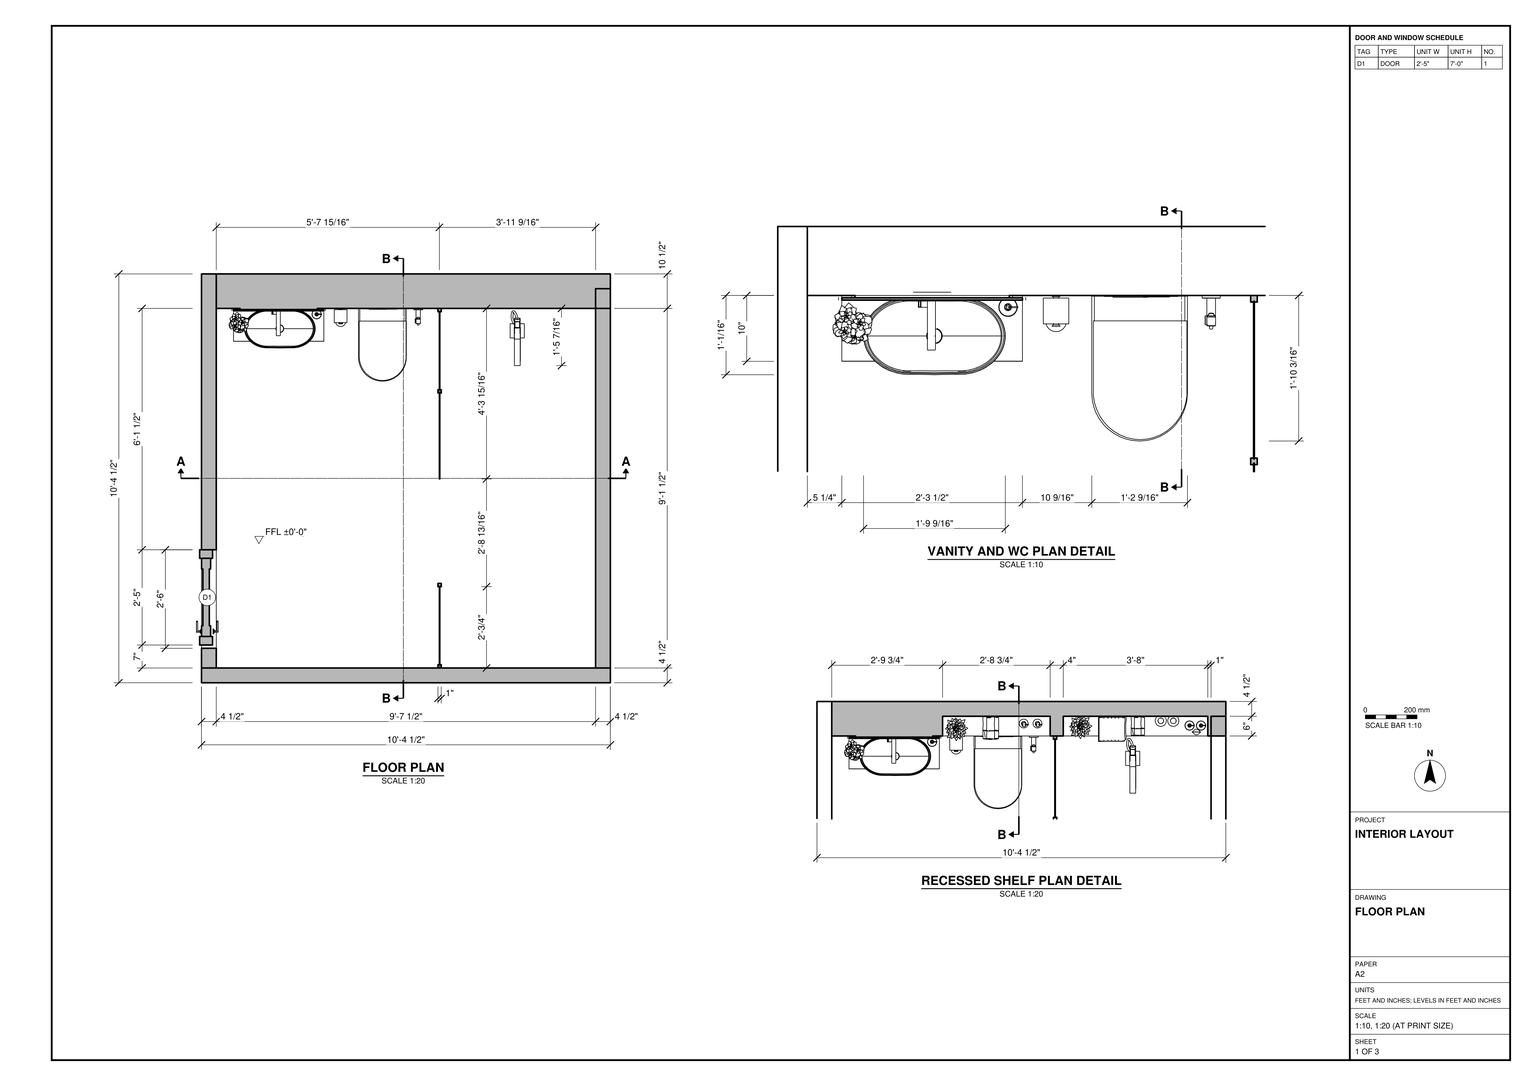
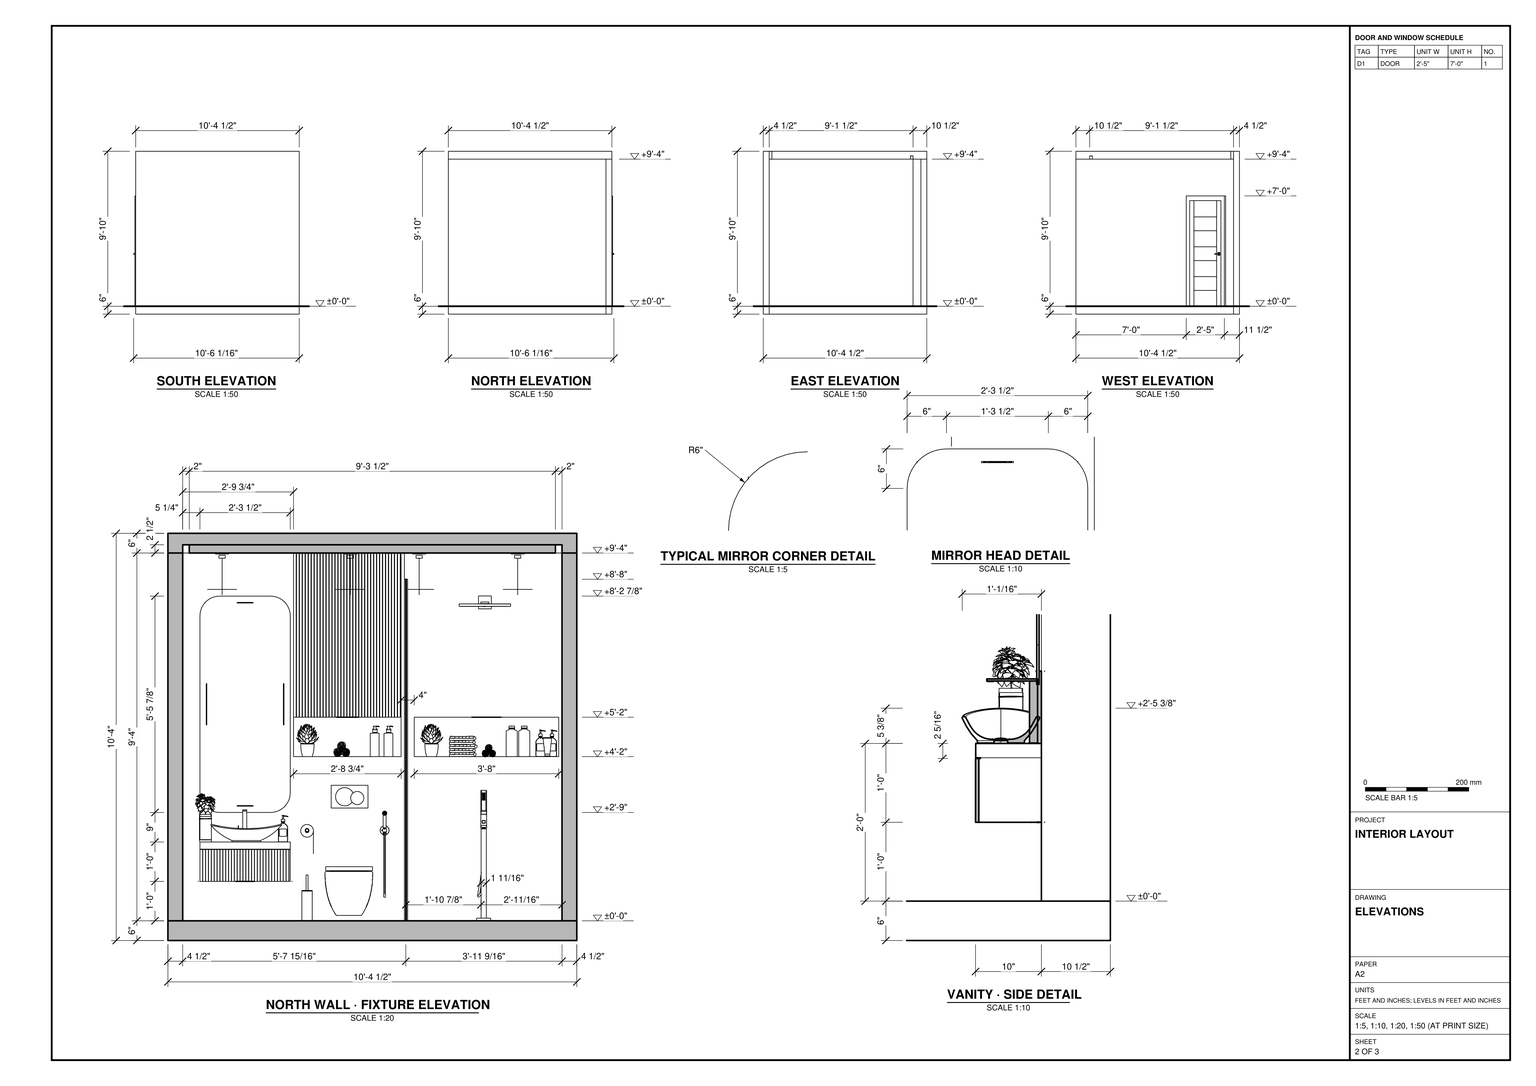
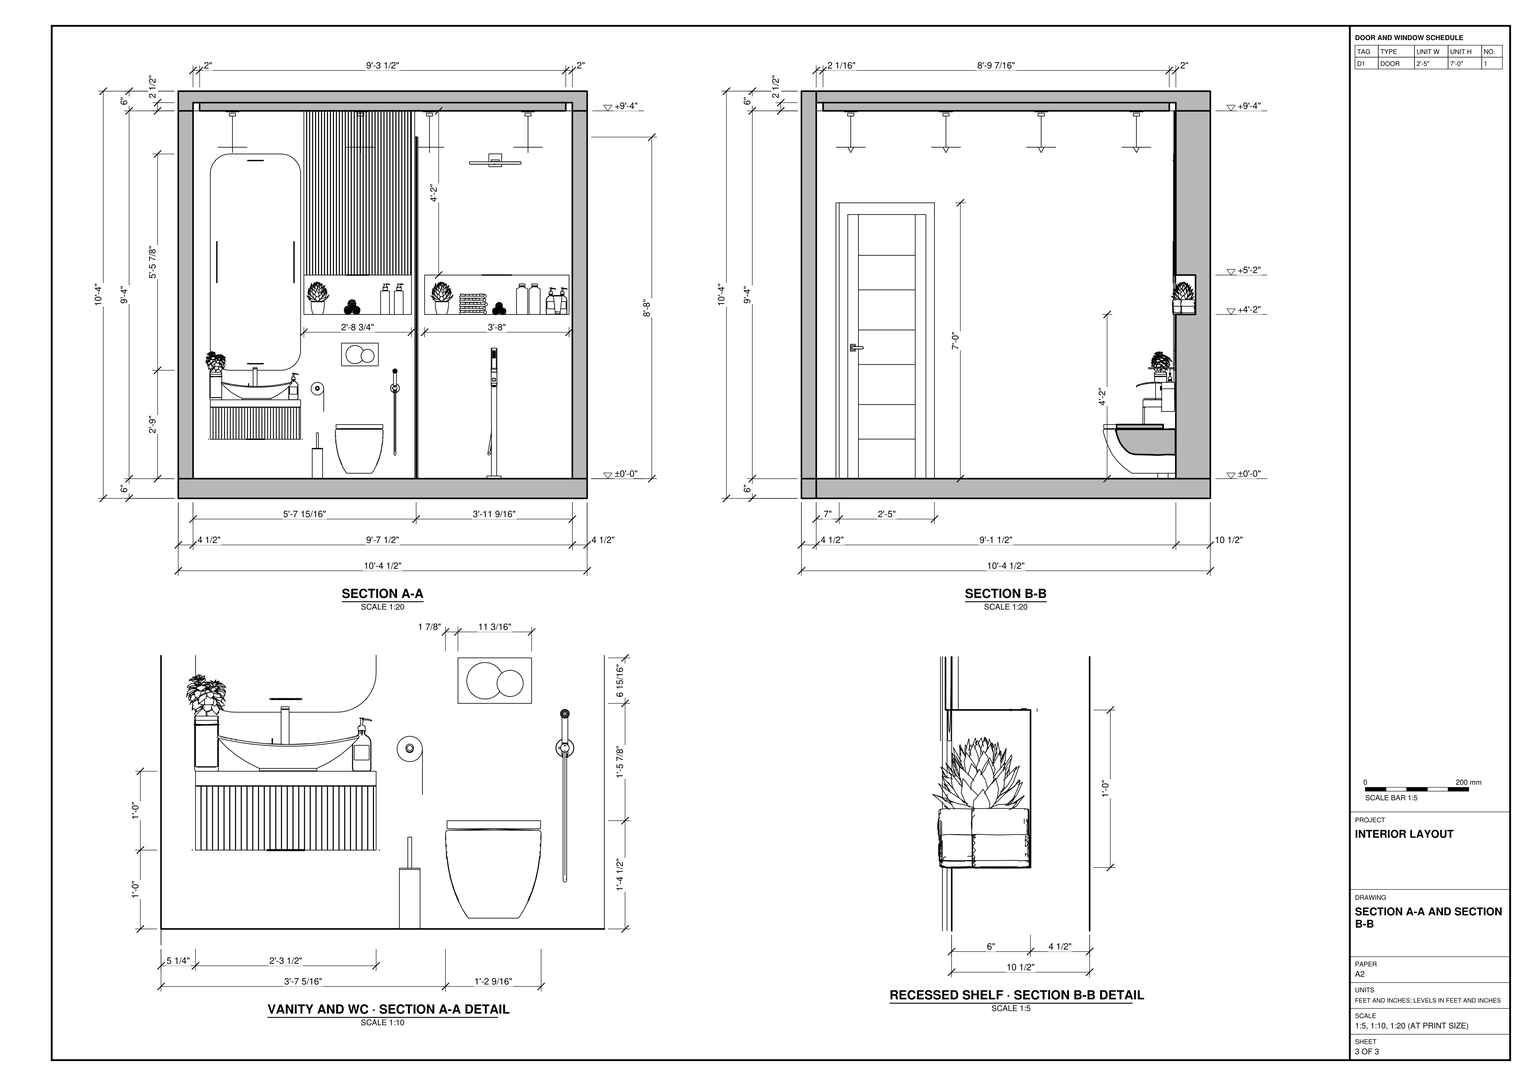
Use the plan, elevations, sections and details in task_files/diagram_01.pdf to build the bathroom in SketchUp. Work in feet and inches. Make the overall model 10'-6 1/16" along X, 10'-4 1/2" along Y and 10'-4" high, with the finished floor at ±0'-0".

Model the floor slab, perimeter walls and ceiling assembly in section. Use the wall thicknesses shown in plan: the north fixture wall is thicker than the other walls to accommodate the recessed shelves. Include the door near the south end of the west wall and a window unit.

Use the north wall elevation to arrange the fixtures. Place the floating vanity with its ribbed front, basin and tap beneath the tall, rounded-corner mirror. Set the wall-hung toilet beside the vanity, with its flush plate above. Model the shelf recesses over the toilet and in the shower area, including the vertically ribbed panel above the toilet recess. On the east side, place the shower fittings behind the glass screens and leave the passage between the screens open as shown in plan. Plants, toiletries, lights and other loose or decorative items may be any suitable library components placed as shown.

Keep the walls, slabs, ceiling assembly and individual fixtures and joinery pieces in separate groups or components. Use components for repeated parts. Save one SketchUp model as output_files/bathroom_with_a_floating_vanity_and_screened_shower.skp.

# SketchUp Ruby script. Lengths in inches.
U = 1.inch
M = Sketchup.active_model
def pt(a) = Geom::Point3d.new(a.map { |v| v * U })
def face(e, loops, mat)
  f = e.add_face(loops[0].map { |a| pt(a) })
  loops[1..].each { |l| e.add_face(l.map { |a| pt(a) }).erase! }
  f.material = f.back_material = mat if mat
  f
end
# faces: each face lists its corners as indices into pts; further lists are holes
def faces(e, pts, list, mat = nil) = list.each { |f| face(e, (f[0].is_a?(Array) ? f : [f]).map { |l| l.map { |i| pts[i] } }, mat) }
# xy, xz, yz: faces in a plane at the given z, y or x. An outline is a flat list of corners, or four numbers for a rectangle; further outlines are holes
def ring(l) = l.size == 4 ? [[l[0], l[1]], [l[2], l[1]], [l[2], l[3]], [l[0], l[3]]] : l.each_slice(2).to_a
def flat(e, list, mat, &to3) = list.each { |f| face(e, (f[0].is_a?(Array) ? f : [f]).map { |l| ring(l).map { |u, v| to3.(u, v) } }, mat) }
def xy(e, z, list, mat = nil) = flat(e, list, mat) { |x, y| [x, y, z] }
def xz(e, y, list, mat = nil) = flat(e, list, mat) { |x, z| [x, y, z] }
def yz(e, x, list, mat = nil) = flat(e, list, mat) { |y, z| [x, y, z] }
def lines(e, pts, list) = list.each { |a, b| e.add_line(pt(pts[a]), pt(pts[b])) }
# prism: a flat outline (further loops are holes) pulled along v
def prism(e, loops, v, mat = nil)
  f = face(e, loops, mat); d = Geom::Vector3d.new(v.map { |x| x * U })
  f.pushpull(f.normal.samedirection?(d) ? d.length : -d.length)
end
def box(e, o, s, mat = nil) = prism(e, [[o, [o[0] + s[0], o[1], o[2]], [o[0] + s[0], o[1] + s[1], o[2]], [o[0], o[1] + s[1], o[2]]]], [0, 0, s[2]], mat)
def at(x, y, z, deg = 0) = Geom::Transformation.translation(pt([x, y, z])) * Geom::Transformation.rotation(ORIGIN, Z_AXIS, deg.degrees)
def axes(o, x, y, z) = Geom::Transformation.new([*x, 0, *y, 0, *z, 0, *pt(o).to_a, 1])
def part(name) = M.definitions.add(name)
# library, detail: a bought-in or finely detailed component or shape, given as its bounding box
def library(name, o, s) = part(name).tap { |d| box(d.entities, o, s) }
def detail(e, o, s) = box(e.add_group.entities, o, s)
def put(e, d, t, mat = nil) = e.add_instance(d, t).tap { |i| i.material = mat if mat }
def group(e, t, mat = nil) = e.add_group.tap { |g| g.transformation = t; g.material = mat if mat }.entities
root = M.entities
M.materials.add("Generic").color = [129, 129, 129]
M.materials["Generic"].alpha = 0.1
M.materials.add("[Color M00]").color = [255, 255, 255]
M.materials.add("[Metal_Corrogated_Shiny]5").color = [193, 193, 193]
M.materials.add("clear glass1").color = [0, 0, 0]
M.materials["clear glass1"].alpha = 0.1
M.materials.add("lz-doorbrown").color = [51, 28, 20]
M.materials.add("lz-doorhandle").color = [114, 114, 114]
c1 = library("lavabo vasque Villeroy",[-11.67,-6.38,0],[23.35,12.76,5.76])
c2 = library("Toilet accessory set",[0,0,0],[28.35,5.51,33.44])
c3 = library("Wall-hung toilet",[0,-0.05,1.64],[14.57,22.16,39.63])
c4 = library("Shower Bath",[-222.28,-28.8,6],[84.83,24.29,98.92])
c5 = library("Potted Basil 50-07",[-3.85,-3.53,0.03],[7.56,8,18.65])
c6 = library("Potted Plant 50-23",[-3.4,-3.5,0],[6.8,7,9.93])
c7 = library("Folded towel stack",[36.8,35.16,1.14],[12.05,13.22,9.67])
c8 = library("Rolled towel stack",[-0.87,0,-0.63],[7.91,9.92,7.86])
c9 = part("Door lever handle")
xy(c9.entities,0,[[0,0,1.888,1.971]])
xy(c9.entities,0.197,[[[0,0,1.888,1.971],[0.307,0.321,1.58,1.65]]])
xy(c9.entities,0.394,[[[0.307,0.321,1.58,1.65],[0.954,0.632,0.96,0.632,0.96,1.339,0.954,1.339,0.868,1.328,0.782,1.292,0.709,1.236,0.653,1.162,0.617,1.077,0.605,0.985,0.617,0.894,0.653,0.808,0.709,0.735,0.782,0.678,0.868,0.643]],[0.954,0.632,0.868,0.643,0.782,0.678,0.709,0.735,0.653,0.808,0.617,0.894,0.605,0.985,0.617,1.077,0.653,1.162,0.709,1.236,0.782,1.292,0.868,1.328,0.954,1.339,0.96,1.339,0.96,0.632],[0.96,0.632,1.265,1.339]])
xy(c9.entities,1.181,[[1.265,0.632,1.265,1.339,4.506,1.339,4.592,1.328,4.677,1.292,4.751,1.236,4.807,1.162,4.842,1.077,4.854,0.985,4.842,0.894,4.807,0.808,4.751,0.735,4.677,0.678,4.592,0.643,4.506,0.632]])
xy(c9.entities,1.535,[[0.954,0.632,0.868,0.643,0.782,0.678,0.709,0.735,0.653,0.808,0.617,0.894,0.605,0.985,0.617,1.077,0.653,1.162,0.709,1.236,0.782,1.292,0.868,1.328,0.954,1.339,4.506,1.339,4.592,1.328,4.677,1.292,4.751,1.236,4.807,1.162,4.842,1.077,4.854,0.985,4.842,0.894,4.807,0.808,4.751,0.735,4.677,0.678,4.592,0.643,4.506,0.632]])
xy(c9.entities,1.575,[[0.956,0.671,0.878,0.681,0.802,0.713,0.737,0.763,0.687,0.828,0.656,0.904,0.645,0.985,0.656,1.067,0.687,1.143,0.737,1.208,0.802,1.258,0.878,1.289,0.956,1.3,4.503,1.3,4.581,1.289,4.657,1.258,4.722,1.208,4.772,1.143,4.804,1.067,4.815,0.985,4.804,0.904,4.772,0.828,4.722,0.763,4.657,0.713,4.581,0.681,4.503,0.671]])
xz(c9.entities,0,[[0,0,1.888,0.197]])
xz(c9.entities,0.321,[[0.307,0.197,1.58,0.394]])
xz(c9.entities,0.632,[[0.954,0.394,0.96,1.535],[0.96,0.394,0.96,1.535,4.506,1.535,4.506,1.181,1.265,1.181,1.265,0.394]])
xz(c9.entities,1.339,[[0.954,0.394,0.96,1.535],[0.96,0.394,1.265,0.394,1.265,1.181,4.506,1.181,4.506,1.535,0.96,1.535]])
xz(c9.entities,1.65,[[0.307,0.197,1.58,0.394]])
xz(c9.entities,1.971,[[0,0,1.888,0.197]])
yz(c9.entities,0,[[0,0,1.971,0.197]])
yz(c9.entities,0.307,[[0.321,0.197,1.65,0.394]])
yz(c9.entities,1.265,[[0.632,0.394,1.339,1.181]])
yz(c9.entities,1.58,[[0.321,0.197,1.65,0.394]])
yz(c9.entities,1.888,[[0,0,1.971,0.197]])
p = [[0.782,0.678,1.535],[0.868,0.643,1.535],[0.868,0.643,0.394],[0.782,0.678,0.394],[0.954,0.632,1.535],[0.954,0.632,0.394],
  [0.653,0.808,1.535],[0.709,0.735,1.535],[0.709,0.735,0.394],[0.653,0.808,0.394],[0.617,0.894,1.535],[0.617,0.894,0.394],
  [0.605,0.985,1.535],[0.605,0.985,0.394],[0.617,1.077,1.535],[0.617,1.077,0.394],[0.653,1.162,1.535],[0.653,1.162,0.394],
  [0.782,1.292,1.535],[0.709,1.236,1.535],[0.709,1.236,0.394],[0.782,1.292,0.394],[0.868,1.328,1.535],[0.868,1.328,0.394],
  [0.954,1.339,1.535],[0.954,1.339,0.394],[4.592,0.643,1.535],[4.506,0.632,1.535],[4.506,0.632,1.181],[4.592,0.643,1.181],
  [4.677,0.678,1.535],[4.677,0.678,1.181],[4.751,0.735,1.535],[4.751,0.735,1.181],[4.807,0.808,1.535],[4.807,0.808,1.181],
  [4.842,0.894,1.535],[4.842,0.894,1.181],[4.854,0.985,1.535],[4.854,0.985,1.181],[4.842,1.077,1.535],[4.842,1.077,1.181],
  [4.807,1.162,1.535],[4.807,1.162,1.181],[4.677,1.292,1.535],[4.751,1.236,1.535],[4.751,1.236,1.181],[4.677,1.292,1.181],
  [4.506,1.339,1.535],[4.592,1.328,1.535],[4.592,1.328,1.181],[4.506,1.339,1.181],[0.802,0.713,1.575],[0.878,0.681,1.575],
  [0.956,0.671,1.575],[0.96,0.632,1.535],[0.96,0.671,1.575],[4.503,0.671,1.575],[4.581,0.681,1.575],[4.657,0.713,1.575],
  [0.687,0.828,1.575],[0.737,0.763,1.575],[4.722,0.763,1.575],[4.772,0.828,1.575],[0.656,0.904,1.575],[4.804,0.904,1.575],
  [0.645,0.985,1.575],[4.815,0.985,1.575],[0.656,1.067,1.575],[4.804,1.067,1.575],[0.687,1.143,1.575],[0.737,1.208,1.575],
  [4.772,1.143,1.575],[4.722,1.208,1.575],[0.802,1.258,1.575],[4.657,1.258,1.575],[0.878,1.289,1.575],[0.956,1.3,1.575],
  [0.96,1.3,1.575],[0.96,1.339,1.535],[4.503,1.3,1.575],[4.581,1.289,1.575]]
faces(c9.entities,p,[[0,1,2,3],[1,4,5,2],[6,7,8,9],[7,0,3,8],[10,6,9,11],[12,10,11,13],[14,12,13,15],[16,14,15,17],
  [18,19,20,21],[19,16,17,20],[22,18,21,23],[24,22,23,25],[26,27,28,29],[30,26,29,31],[32,30,31,33],[34,32,33,35],
  [36,34,35,37],[38,36,37,39],[40,38,39,41],[42,40,41,43],[44,45,46,47],[45,42,43,46],[48,49,50,51],[49,44,47,50],
  [0,52,53,1],[1,53,54,4],[55,56,57,27],[54,56,55,4],[27,57,58,26],[26,58,59,30],[6,60,61,7],[7,61,52,0],
  [30,59,62,32],[32,62,63,34],[10,64,60,6],[34,63,65,36],[12,66,64,10],[36,65,67,38],[14,68,66,12],[38,67,69,40],
  [16,70,68,14],[19,71,70,16],[42,72,73,45],[40,69,72,42],[18,74,71,19],[45,73,75,44],[22,76,74,18],[24,77,76,22],
  [78,77,24,79],[79,48,80,78],[49,81,80,48],[44,75,81,49]])
c10 = part("door by lz")
put(c10.entities,c9,axes([9.99,-3.35,36.38],[1,0,0],[0,0,1],[0,-1,0]),"lz-doorhandle")
put(c10.entities,c9,axes([10.03,0.12,36.38],[1,0,0],[0,0,1],[0,1,0]),"lz-doorhandle")
g1 = group(c10.entities,at(5.91,0,0),"lz-doorbrown")
prism(g1,[[[35.43,0,0],[32.26,0,0],[32.26,0,75.4],[3.18,0,75.4],[3.18,0,0],[0,0,0],[0,0,78.74],[35.43,0,78.74]]],[0,-3.9375,0])
g2 = group(c10.entities,at(9.09,-0.59,0),"lz-doorbrown")
xy(g2,0,[[0,-2.76,3.97,-2.76,3.97,-2.36,25.11,-2.36,25.11,-2.76,29.08,-2.76,29.08,0,25.11,0,25.11,-0.39,3.97,-0.39,3.97,0,0,0]])
xy(g2,11.29,[[3.97,-2.36,25.11,-1.97],[3.97,-0.79,25.11,-0.39]])
xy(g2,21.14,[[3.97,-2.36,25.11,-1.97],[3.97,-0.79,25.11,-0.39]])
xy(g2,32.6,[[3.97,-2.36,25.11,-1.97],[3.97,-0.79,25.11,-0.39]])
xy(g2,42.45,[[3.97,-2.36,25.11,-1.97],[3.97,-0.79,25.11,-0.39]])
xy(g2,53.9,[[3.97,-2.36,25.11,-1.97],[3.97,-0.79,25.11,-0.39]])
xy(g2,63.75,[[3.97,-2.36,25.11,-1.97],[3.97,-0.79,25.11,-0.39]])
xy(g2,75.4,[[0,-2.76,0,0,3.97,0,3.97,-0.39,25.11,-0.39,25.11,0,29.08,0,29.08,-2.76,25.11,-2.76,25.11,-2.36,3.97,-2.36,3.97,-2.76]])
xz(g2,-2.76,[[0,0,3.97,75.4],[25.11,0,29.08,75.4]])
xz(g2,-2.36,[[3.97,0,25.11,11.29],[3.97,21.14,25.11,32.6],[3.97,42.45,25.11,53.9],[3.97,63.75,25.11,75.4]])
xz(g2,-1.97,[[3.97,11.29,25.11,21.14],[3.97,32.6,25.11,42.45],[3.97,53.9,25.11,63.75]])
xz(g2,-0.79,[[3.97,11.29,25.11,21.14],[3.97,32.6,25.11,42.45],[3.97,53.9,25.11,63.75]])
xz(g2,-0.39,[[3.97,0,25.11,11.29],[3.97,21.14,25.11,32.6],[3.97,42.45,25.11,53.9],[3.97,63.75,25.11,75.4]])
xz(g2,0,[[0,0,3.97,75.4],[25.11,0,29.08,75.4]])
yz(g2,0,[[-2.76,0,0,75.4]])
yz(g2,3.97,[[-2.76,0,-2.76,75.4,-2.36,75.4,-2.36,63.75,-1.97,63.75,-1.97,53.9,-2.36,53.9,-2.36,42.45,-1.97,42.45,-1.97,32.6,-2.36,32.6,-2.36,21.14,-1.97,21.14,-1.97,11.29,-2.36,11.29,-2.36,0],[-0.39,0,-0.39,11.29,-0.79,11.29,-0.79,21.14,-0.39,21.14,-0.39,32.6,-0.79,32.6,-0.79,42.45,-0.39,42.45,-0.39,53.9,-0.79,53.9,-0.79,63.75,-0.39,63.75,-0.39,75.4,0,75.4,0,0]])
yz(g2,25.11,[[-2.76,0,-2.36,0,-2.36,11.29,-1.97,11.29,-1.97,21.14,-2.36,21.14,-2.36,32.6,-1.97,32.6,-1.97,42.45,-2.36,42.45,-2.36,53.9,-1.97,53.9,-1.97,63.75,-2.36,63.75,-2.36,75.4,-2.76,75.4],[-0.39,0,0,0,0,75.4,-0.39,75.4,-0.39,63.75,-0.79,63.75,-0.79,53.9,-0.39,53.9,-0.39,42.45,-0.79,42.45,-0.79,32.6,-0.39,32.6,-0.39,21.14,-0.79,21.14,-0.79,11.29,-0.39,11.29]])
yz(g2,29.08,[[-2.76,0,0,75.4]])
c11 = part("Group7\#1")
box(c11.entities,[-16.375,-25,0],[0.79,50,0.47])
c12 = part("Group8\#1")
box(c12.entities,[-15.47,-25,0],[0.79,50,0.47])
c13 = part("Group9\#1")
box(c13.entities,[-14.5625,-25,0],[0.78,50,0.47])
c14 = part("Group10\#1")
box(c14.entities,[-13.66,-25,0],[0.79,50,0.47])
c15 = part("Group11\#1")
box(c15.entities,[-12.75,-25,0],[0.78,50,0.47])
c16 = part("Group12\#1")
box(c16.entities,[-11.85,-25,0],[0.79,50,0.47])
c17 = part("Group13\#1")
box(c17.entities,[-10.94,-25,0],[0.79,50,0.47])
c18 = part("Group14\#1")
box(c18.entities,[-10.04,-25,0],[0.79,50,0.47])
c19 = part("Group15\#1")
box(c19.entities,[-9.13,-25,0],[0.79,50,0.47])
c20 = part("Group16\#1")
box(c20.entities,[-8.23,-25,0],[0.79,50,0.47])
c21 = part("Group17\#1")
box(c21.entities,[-7.32,-25,0],[0.79,50,0.47])
c22 = part("Group18\#1")
box(c22.entities,[-6.41,-25,0],[0.79,50,0.47])
c23 = part("Group19\#1")
box(c23.entities,[-5.51,-25,0],[0.79,50,0.47])
c24 = part("Group20\#1")
box(c24.entities,[-4.6,-25,0],[0.78,50,0.47])
c25 = part("Group21\#1")
box(c25.entities,[-3.7,-25,0],[0.79,50,0.47])
c26 = part("Group22\#1")
box(c26.entities,[-2.79,-25,0],[0.79,50,0.47])
c27 = part("Group23\#1")
box(c27.entities,[-1.89,-25,0],[0.79,50,0.47])
c28 = part("Group24\#1")
box(c28.entities,[-0.98,-25,0],[0.79,50,0.47])
c29 = part("Group25\#1")
box(c29.entities,[-0.08,-25,0],[0.79,50,0.47])
c30 = part("Group26\#1")
box(c30.entities,[0.83,-25,0],[0.79,50,0.47])
c31 = part("Group27\#1")
box(c31.entities,[1.74,-25,0],[0.78,50,0.47])
c32 = part("Group28\#1")
box(c32.entities,[2.64,-25,0],[0.79,50,0.47])
c33 = part("Group29\#1")
box(c33.entities,[3.55,-25,0],[0.78,50,0.47])
c34 = part("Group30\#1")
box(c34.entities,[4.45,-25,0],[0.79,50,0.47])
c35 = part("Group31\#1")
box(c35.entities,[5.36,-25,0],[0.78,50,0.47])
c36 = part("Group32\#1")
box(c36.entities,[6.26,-25,0],[0.79,50,0.47])
c37 = part("Group33\#1")
box(c37.entities,[7.17,-25,0],[0.79,50,0.47])
c38 = part("Group34\#1")
box(c38.entities,[8.07,-25,0],[0.79,50,0.47])
c39 = part("Group35\#1")
box(c39.entities,[8.98,-25,0],[0.79,50,0.47])
c40 = part("Group36\#1")
box(c40.entities,[9.88,-25,0],[0.79,50,0.47])
c41 = part("Group37\#1")
box(c41.entities,[10.79,-25,0],[0.79,50,0.47])
c42 = part("Group38\#1")
box(c42.entities,[11.7,-25,0],[0.78,50,0.47])
c43 = part("Group39\#1")
box(c43.entities,[12.6,-25,0],[0.79,50,0.47])
c44 = part("Group40\#1")
box(c44.entities,[13.51,-25,0],[0.78,50,0.47])
c45 = part("Group41\#1")
box(c45.entities,[14.41,-25,0],[0.79,50,0.47])
c46 = part("Group42\#1")
box(c46.entities,[15.32,-25,0],[0.79,50,0.47])
c47 = part("Group43\#1")
xy(c47.entities,0,[[16.22,-25,16.375,25]])
xy(c47.entities,0.47,[[16.22,-25,16.375,25]])
yz(c47.entities,16.22,[[-25,0,25,0.47]])
c48 = part("Group5\#1")
put(c48.entities,c11,at(0,0,0))
put(c48.entities,c12,at(0,0,0))
put(c48.entities,c13,at(0,0,0))
put(c48.entities,c14,at(0,0,0))
put(c48.entities,c15,at(0,0,0))
put(c48.entities,c16,at(0,0,0))
put(c48.entities,c17,at(0,0,0))
put(c48.entities,c18,at(0,0,0))
put(c48.entities,c19,at(0,0,0))
put(c48.entities,c20,at(0,0,0))
put(c48.entities,c21,at(0,0,0))
put(c48.entities,c22,at(0,0,0))
put(c48.entities,c23,at(0,0,0))
put(c48.entities,c24,at(0,0,0))
put(c48.entities,c25,at(0,0,0))
put(c48.entities,c26,at(0,0,0))
put(c48.entities,c27,at(0,0,0))
put(c48.entities,c28,at(0,0,0))
put(c48.entities,c29,at(0,0,0))
put(c48.entities,c30,at(0,0,0))
put(c48.entities,c31,at(0,0,0))
put(c48.entities,c32,at(0,0,0))
put(c48.entities,c33,at(0,0,0))
put(c48.entities,c34,at(0,0,0))
put(c48.entities,c35,at(0,0,0))
put(c48.entities,c36,at(0,0,0))
put(c48.entities,c37,at(0,0,0))
put(c48.entities,c38,at(0,0,0))
put(c48.entities,c39,at(0,0,0))
put(c48.entities,c40,at(0,0,0))
put(c48.entities,c41,at(0,0,0))
put(c48.entities,c42,at(0,0,0))
put(c48.entities,c43,at(0,0,0))
put(c48.entities,c44,at(0,0,0))
put(c48.entities,c45,at(0,0,0))
put(c48.entities,c46,at(0,0,0))
put(c48.entities,c47,at(0,0,0))
c49 = part("Group46\#1")
box(c49.entities,[-13.75,-4.85,0],[0.8125,9.7,0.5])
c50 = part("Group47\#1")
box(c50.entities,[-12.875,-4.85,0],[0.8125,9.7,0.5])
c51 = part("Group48\#1")
box(c51.entities,[-12,-4.85,0],[0.8125,9.7,0.5])
c52 = part("Group49\#1")
box(c52.entities,[-11.125,-4.85,0],[0.8125,9.7,0.5])
c53 = part("Group50\#1")
box(c53.entities,[-10.25,-4.85,0],[0.8125,9.7,0.5])
c54 = part("Group51\#1")
box(c54.entities,[-9.375,-4.85,0],[0.8125,9.7,0.5])
c55 = part("Group52\#1")
box(c55.entities,[-8.5,-4.85,0],[0.8125,9.7,0.5])
c56 = part("Group53\#1")
box(c56.entities,[-7.625,-4.85,0],[0.8125,9.7,0.5])
c57 = part("Group54\#1")
box(c57.entities,[-6.75,-4.85,0],[0.8125,9.7,0.5])
c58 = part("Group55\#1")
box(c58.entities,[-5.875,-4.85,0],[0.8125,9.7,0.5])
c59 = part("Group56\#1")
box(c59.entities,[-5,-4.85,0],[0.8125,9.7,0.5])
c60 = part("Group57\#1")
box(c60.entities,[-4.125,-4.85,0],[0.8125,9.7,0.5])
c61 = part("Group58\#1")
box(c61.entities,[-3.25,-4.85,0],[0.8125,9.7,0.5])
c62 = part("Group59\#1")
box(c62.entities,[-2.375,-4.85,0],[0.8125,9.7,0.5])
c63 = part("Group60\#1")
box(c63.entities,[-1.5,-4.85,0],[0.8125,9.7,0.5])
c64 = part("Group61\#1")
box(c64.entities,[-0.625,-4.85,0],[0.8125,9.7,0.5])
c65 = part("Group62\#1")
box(c65.entities,[0.25,-4.85,0],[0.8125,9.7,0.5])
c66 = part("Group63\#1")
box(c66.entities,[1.125,-4.85,0],[0.8125,9.7,0.5])
c67 = part("Group64\#1")
box(c67.entities,[2,-4.85,0],[0.8125,9.7,0.5])
c68 = part("Group65\#1")
box(c68.entities,[2.875,-4.85,0],[0.8125,9.7,0.5])
c69 = part("Group66\#1")
box(c69.entities,[3.75,-4.85,0],[0.8125,9.7,0.5])
c70 = part("Group67\#1")
box(c70.entities,[4.625,-4.85,0],[0.8125,9.7,0.5])
c71 = part("Group68\#1")
box(c71.entities,[5.5,-4.85,0],[0.8125,9.7,0.5])
c72 = part("Group69\#1")
box(c72.entities,[6.375,-4.85,0],[0.8125,9.7,0.5])
c73 = part("Group70\#1")
box(c73.entities,[7.25,-4.85,0],[0.8125,9.7,0.5])
c74 = part("Group71\#1")
box(c74.entities,[8.125,-4.85,0],[0.8125,9.7,0.5])
c75 = part("Group72\#1")
box(c75.entities,[9,-4.85,0],[0.8125,9.7,0.5])
c76 = part("Group73\#1")
box(c76.entities,[9.875,-4.85,0],[0.8125,9.7,0.5])
c77 = part("Group74\#1")
box(c77.entities,[10.75,-4.85,0],[0.8125,9.7,0.5])
c78 = part("Group75\#1")
box(c78.entities,[11.625,-4.85,0],[0.8125,9.7,0.5])
c79 = part("Group76\#1")
box(c79.entities,[12.5,-4.85,0],[0.8125,9.7,0.5])
c80 = part("Group77\#1")
box(c80.entities,[13.375,-4.85,0],[0.375,9.7,0.5])
c81 = part("Group44\#1")
put(c81.entities,c49,at(0,0,0))
put(c81.entities,c50,at(0,0,0))
put(c81.entities,c51,at(0,0,0))
put(c81.entities,c52,at(0,0,0))
put(c81.entities,c53,at(0,0,0))
put(c81.entities,c54,at(0,0,0))
put(c81.entities,c55,at(0,0,0))
put(c81.entities,c56,at(0,0,0))
put(c81.entities,c57,at(0,0,0))
put(c81.entities,c58,at(0,0,0))
put(c81.entities,c59,at(0,0,0))
put(c81.entities,c60,at(0,0,0))
put(c81.entities,c61,at(0,0,0))
put(c81.entities,c62,at(0,0,0))
put(c81.entities,c63,at(0,0,0))
put(c81.entities,c64,at(0,0,0))
put(c81.entities,c65,at(0,0,0))
put(c81.entities,c66,at(0,0,0))
put(c81.entities,c67,at(0,0,0))
put(c81.entities,c68,at(0,0,0))
put(c81.entities,c69,at(0,0,0))
put(c81.entities,c70,at(0,0,0))
put(c81.entities,c71,at(0,0,0))
put(c81.entities,c72,at(0,0,0))
put(c81.entities,c73,at(0,0,0))
put(c81.entities,c74,at(0,0,0))
put(c81.entities,c75,at(0,0,0))
put(c81.entities,c76,at(0,0,0))
put(c81.entities,c77,at(0,0,0))
put(c81.entities,c78,at(0,0,0))
put(c81.entities,c79,at(0,0,0))
put(c81.entities,c80,at(0,0,0))
c82 = library("Group\#18",[-0.5,-0.5,-0.1],[28.5,2,0.2])
c83 = library("Group\#5",[-0.5,-0.5,-0.1],[24.5,1.35,0.2])
c84 = library("Group\#6",[-0.5,-0.5,0],[1,1.35,61.875])
c85 = library("Group\#7",[-0.5,-0.5,-0.1],[24.5,1.35,0.2])
c86 = library("Group\#8",[-0.5,-0.5,0],[1,1.35,61.875])
c87 = part("Grupo\#1")
xy(c87.entities,0,[[[0,7.8,1.8125,9.61],[0.16,7.95,1.65,9.45]]],"[Metal_Corrogated_Shiny]5")
xy(c87.entities,0.08,[[[0,7.8,1.8125,9.61],[0.16,7.95,1.65,9.45]],[0.16,7.95,1.65,9.45]],"[Metal_Corrogated_Shiny]5")
xy(c87.entities,3.23,[[1.65,7.95,2.83,9.45],[2.95,7.95,3.35,9.45]],"[Metal_Corrogated_Shiny]5")
xy(c87.entities,3.31,[[2.83,8.03,2.95,9.37]],"[Metal_Corrogated_Shiny]5")
xy(c87.entities,4.65,[[2.83,8.03,2.95,9.37]],"[Metal_Corrogated_Shiny]5")
xy(c87.entities,4.72,[[1.65,7.95,2.83,9.45],[2.95,7.95,3.23,9.45]],"[Metal_Corrogated_Shiny]5")
xy(c87.entities,6.1,[[3.23,7.95,3.35,9.45]],"[Metal_Corrogated_Shiny]5")
xy(c87.entities,11.5,[[[0.16,7.95,1.65,9.45],[0.89,8.03,0.72,8.06,0.56,8.13,0.42,8.24,0.32,8.38,0.26,8.54,0.24,8.71,0.26,8.89,0.33,9.05,0.44,9.18,0.58,9.29,0.74,9.35,0.92,9.37,1.09,9.34,1.25,9.27,1.39,9.16,1.49,9.02,1.56,8.86,1.57,8.6875,1.55,8.52,1.48,8.35,1.37,8.22,1.23,8.11,1.07,8.05]]],"[Metal_Corrogated_Shiny]5")
xy(c87.entities,11.54,[[0.91,0.12,0.75,0.14,0.61,0.2,0.49,0.29,0.39,0.41,0.36,0.48,0.34,0.56,0.31,0.71,0.34,0.86,0.39,1,0.49,1.125,0.61,1.22,0.75,1.28,0.91,1.3,1.06,1.28,1.2,1.22,1.32,1.125,1.42,1,1.48,0.86,1.5,0.71,1.48,0.56,1.42,0.41,1.32,0.29,1.2,0.2,1.06,0.14]],"[Metal_Corrogated_Shiny]5")
xy(c87.entities,11.61,[[[0.22,0,0.18,0.02,0.16,0.06,0.16,9.39,0.18,9.43,0.2,9.4375,0.22,9.45,1.6,9.45,1.61,9.4375,1.63,9.43,1.65,9.39,1.65,0.06,1.63,0.02,1.61,0.01,1.6,0],[0.91,0.12,1.06,0.14,1.2,0.2,1.32,0.29,1.42,0.41,1.48,0.56,1.5,0.71,1.48,0.86,1.42,1,1.32,1.125,1.2,1.22,1.06,1.28,0.91,1.3,0.75,1.28,0.61,1.22,0.49,1.125,0.39,1,0.34,0.86,0.31,0.71,0.34,0.56,0.36,0.48,0.39,0.41,0.49,0.29,0.61,0.2,0.75,0.14]],[0.91,0.12,0.75,0.14,0.61,0.2,0.49,0.29,0.39,0.41,0.36,0.48,0.34,0.56,0.31,0.71,0.34,0.86,0.39,1,0.49,1.125,0.61,1.22,0.75,1.28,0.91,1.3,1.06,1.28,1.2,1.22,1.32,1.125,1.42,1,1.48,0.86,1.5,0.71,1.48,0.56,1.42,0.41,1.32,0.29,1.2,0.2,1.06,0.14],[0.89,8.03,1.07,8.05,1.23,8.11,1.37,8.22,1.48,8.35,1.55,8.52,1.57,8.6875,1.56,8.86,1.49,9.02,1.39,9.16,1.25,9.27,1.09,9.34,0.92,9.37,0.74,9.35,0.58,9.29,0.44,9.18,0.33,9.05,0.26,8.89,0.24,8.71,0.26,8.54,0.32,8.38,0.42,8.24,0.56,8.13,0.72,8.06]],"[Metal_Corrogated_Shiny]5")
xy(c87.entities,12.01,[[0.22,0,0.18,0.02,0.16,0.06,0.16,9.39,0.18,9.43,0.2,9.4375,0.22,9.45,1.6,9.45,1.61,9.4375,1.63,9.43,1.65,9.39,1.65,0.06,1.63,0.02,1.61,0.01,1.6,0]],"[Metal_Corrogated_Shiny]5")
xz(c87.entities,0,[[0.22,11.61,0.24,12.01],[0.24,11.61,1.57,12.01],[1.57,11.61,1.6,12.01]],"[Metal_Corrogated_Shiny]5")
xz(c87.entities,7.8,[[0,0,1.8125,0.08]],"[Metal_Corrogated_Shiny]5")
xz(c87.entities,7.95,[[0.16,0,1.65,0.08],[0.16,0.08,1.65,0.08,1.65,3.23,2.83,3.23,2.83,4.72,1.65,4.72,1.65,11.5,0.16,11.5],[2.95,3.23,3.35,3.23,3.35,6.1,3.23,6.1,3.23,4.72,2.95,4.72]],"[Metal_Corrogated_Shiny]5")
xz(c87.entities,8.03,[[2.83,3.31,2.95,4.65]],"[Metal_Corrogated_Shiny]5")
xz(c87.entities,9.37,[[2.83,3.31,2.95,4.65]],"[Metal_Corrogated_Shiny]5")
xz(c87.entities,9.45,[[0.16,0,1.65,0.08],[0.16,0.08,0.16,11.5,1.65,11.5,1.65,4.72,2.83,4.72,2.83,3.23,1.65,3.23,1.65,0.08],[2.95,3.23,2.95,4.72,3.23,4.72,3.23,6.1,3.35,6.1,3.35,3.23],[0.22,11.61,0.24,12.01],[0.24,11.61,1.57,12.01],
  [1.57,11.61,1.6,12.01]],"[Metal_Corrogated_Shiny]5")
xz(c87.entities,9.61,[[0,0,1.8125,0.08]],"[Metal_Corrogated_Shiny]5")
yz(c87.entities,0,[[7.8,0,9.61,0.08]],"[Metal_Corrogated_Shiny]5")
yz(c87.entities,0.16,[[7.95,0,9.45,0.08],[7.95,0.08,9.45,11.5],[0.06,11.61,0.08,12.01],[0.08,11.61,9.37,12.01],[9.37,11.61,9.39,12.01]],"[Metal_Corrogated_Shiny]5")
yz(c87.entities,1.65,[[7.95,0,9.45,0.08],[7.95,0.08,9.45,3.23],[7.95,4.72,9.45,11.5],[0.06,11.61,0.08,12.01],[0.08,11.61,9.37,12.01],
  [9.37,11.61,9.39,12.01]],"[Metal_Corrogated_Shiny]5")
yz(c87.entities,1.8125,[[7.8,0,9.61,0.08]],"[Metal_Corrogated_Shiny]5")
yz(c87.entities,2.83,[[[7.95,3.23,9.45,4.72],[8.03,3.31,9.37,4.65]]],"[Metal_Corrogated_Shiny]5")
yz(c87.entities,2.95,[[[7.95,3.23,9.45,4.72],[8.03,3.31,9.37,4.65]],[8.03,3.31,9.37,4.65]],"[Metal_Corrogated_Shiny]5")
yz(c87.entities,3.23,[[7.95,4.72,9.45,6.1]],"[Metal_Corrogated_Shiny]5")
yz(c87.entities,3.35,[[7.95,3.23,9.45,6.1]],"[Metal_Corrogated_Shiny]5")
p = [[0.75,0.14,11.61],[0.61,0.2,11.61],[0.61,0.2,11.54],[0.75,0.14,11.54],[0.91,0.12,11.61],[0.91,0.12,11.54],
  [1.06,0.14,11.61],[1.06,0.14,11.54],[1.2,0.2,11.61],[1.2,0.2,11.54],[0.49,0.29,11.61],[0.49,0.29,11.54],
  [1.32,0.29,11.61],[1.32,0.29,11.54],[0.39,0.41,11.61],[0.39,0.41,11.54],[1.42,0.41,11.61],[1.42,0.41,11.54],
  [0.36,0.48,11.61],[0.36,0.48,11.54],[1.48,0.56,11.61],[1.48,0.56,11.54],[0.34,0.56,11.61],[0.34,0.56,11.54],
  [0.31,0.71,11.61],[0.31,0.71,11.54],[1.5,0.71,11.61],[1.5,0.71,11.54],[0.34,0.86,11.61],[0.34,0.86,11.54],
  [1.48,0.86,11.61],[1.48,0.86,11.54],[0.39,1,11.61],[0.39,1,11.54],[1.42,1,11.61],[1.42,1,11.54],
  [0.49,1.125,11.61],[0.49,1.125,11.54],[1.32,1.125,11.61],[1.32,1.125,11.54],[0.61,1.22,11.61],[0.61,1.22,11.54],
  [1.2,1.22,11.61],[1.2,1.22,11.54],[0.75,1.28,11.61],[0.75,1.28,11.54],[1.06,1.28,11.61],[1.06,1.28,11.54],
  [0.91,1.3,11.61],[0.91,1.3,11.54],[0.72,8.06,11.5],[0.89,8.03,11.5],[0.89,8.03,11.61],[0.72,8.06,11.61],
  [1.07,8.05,11.5],[1.07,8.05,11.61],[0.42,8.24,11.5],[0.56,8.13,11.5],[0.56,8.13,11.61],[0.42,8.24,11.61],
  [1.23,8.11,11.5],[1.23,8.11,11.61],[1.37,8.22,11.5],[1.37,8.22,11.61],[0.32,8.38,11.5],[0.32,8.38,11.61],
  [1.48,8.35,11.5],[1.48,8.35,11.61],[0.26,8.54,11.5],[0.26,8.54,11.61],[1.55,8.52,11.5],[1.55,8.52,11.61],
  [0.24,8.71,11.5],[0.24,8.71,11.61],[1.57,8.6875,11.5],[1.57,8.6875,11.61],[0.26,8.89,11.5],[0.26,8.89,11.61],
  [1.56,8.86,11.5],[1.56,8.86,11.61],[0.33,9.05,11.5],[0.33,9.05,11.61],[1.49,9.02,11.5],[1.49,9.02,11.61],
  [0.44,9.18,11.5],[0.44,9.18,11.61],[1.39,9.16,11.5],[1.39,9.16,11.61],[0.58,9.29,11.5],[0.58,9.29,11.61],
  [1.25,9.27,11.5],[1.25,9.27,11.61],[0.74,9.35,11.5],[0.74,9.35,11.61],[1.09,9.34,11.5],[0.92,9.37,11.5],
  [0.92,9.37,11.61],[1.09,9.34,11.61],[0.18,0.02,11.61],[0.18,0.02,12.01],[0.17,0.04,12.01],[0.17,0.04,11.61],
  [0.22,0,11.61],[0.22,0,12.01],[0.2,0.01,12.01],[0.2,0.01,11.61],[0.16,0.06,12.01],[0.16,0.06,11.61],
  [1.63,0.02,11.61],[1.63,0.02,12.01],[1.61,0.01,12.01],[1.61,0.01,11.61],[1.65,0.06,11.61],[1.65,0.06,12.01],
  [1.64,0.04,12.01],[1.64,0.04,11.61],[1.6,0,12.01],[1.6,0,11.61],[0.22,9.45,12.01],[0.22,9.45,11.61],
  [0.2,9.4375,11.61],[0.2,9.4375,12.01],[0.18,9.43,11.61],[0.18,9.43,12.01],[0.17,9.41,12.01],[0.17,9.41,11.61],
  [0.16,9.39,11.61],[0.16,9.39,12.01],[1.61,9.4375,11.61],[1.61,9.4375,12.01],[1.63,9.43,12.01],[1.63,9.43,11.61],
  [1.64,9.41,12.01],[1.64,9.41,11.61],[1.65,9.39,12.01],[1.65,9.39,11.61],[1.6,9.45,11.61],[1.6,9.45,12.01],
  [2.95,8.03,3.31],[3.35,8.03,3.31],[2.95,8.03,4.65],[3.35,8.03,4.65],[2.95,9.37,3.31],[3.35,9.37,3.31],
  [2.95,9.37,4.65],[3.35,9.37,4.65]]
faces(c87.entities,p,[[0,1,2,3],[4,0,3,5],[6,4,5,7],[8,6,7,9],[1,10,11,2],[12,8,9,13],[10,14,15,11],[16,12,13,17],
  [14,18,19,15],[20,16,17,21],[18,22,23,19],[22,24,25,23],[26,20,21,27],[24,28,29,25],[30,26,27,31],[28,32,33,29],
  [34,30,31,35],[32,36,37,33],[38,34,35,39],[36,40,41,37],[42,38,39,43],[40,44,45,41],[46,42,43,47],[44,48,49,45],
  [48,46,47,49],[50,51,52,53],[51,54,55,52],[56,57,58,59],[57,50,53,58],[54,60,61,55],[60,62,63,61],[64,56,59,65],
  [62,66,67,63],[68,64,65,69],[66,70,71,67],[72,68,69,73],[70,74,75,71],[76,72,73,77],[74,78,79,75],[80,76,77,81],
  [78,82,83,79],[84,80,81,85],[82,86,87,83],[88,84,85,89],[86,90,91,87],[92,88,89,93],[94,95,96,97],[90,94,97,91],
  [95,92,93,96],[98,99,100,101],[102,103,104,105],[105,104,99,98],[101,100,106,107],[108,109,110,111],[112,113,114,115],[115,114,109,108],
  [111,110,116,117],[118,119,120,121],[121,120,122,123],[124,125,126,127],[123,122,125,124],[128,129,130,131],[131,130,132,133],[133,132,134,135],
  [136,137,129,128]],"[Metal_Corrogated_Shiny]5")
lines(c87.entities,p,[[138,139],[140,141],[142,143],[144,145]])
c88 = part("Group\#10")
box(c88.entities,[0,-24,0],[0.12,24,104])
c89 = library("Group\#16",[-0.5,-0.5,-0.1],[45,1.98,0.2])
c90 = library("Group\#17",[-0.5,-0.5,-0.1],[33.75,2,0.2])
c91 = library("Group\#21",[-0.5,-0.5,-0.1],[3,106.42,0.2])
c92 = library("Group\#22",[-0.5,-0.5,-0.1],[116.5,3,0.2])
c93 = library("Group\#23",[-0.5,-0.5,-0.1],[3,106.42,0.2])
c94 = library("Group\#24",[-0.5,-0.5,-0.1],[116.5,3.08,0.2])
c95 = library("Group\#26",[0,0,0],[8.9,8.9,12.71])
xy(root,6,[[6.05,114,126.05,124.5]])
xy(root,56,[[39.8,114,72.55,120],[76.55,114,120.55,120]])
xy(root,68,[[39.8,114,72.55,119],[76.55,114,120.55,119.02]])
xy(root,118,[[6.05,114,126.05,124.5]])
xz(root,114,[[[6.05,6,73.55,6,73.55,118,72.55,118,72.55,56,39.8,56,39.8,118,6.05,118],[13.3,41,36.8,102.875]],[[73.55,6,126.05,118],[76.55,56,120.55,68]]])
xz(root,120,[[39.8,56,72.55,68],[76.55,56,120.55,68]])
xz(root,124.5,[[6.05,6,126.05,118]])
yz(root,6.05,[[114,6,124.5,118]])
yz(root,39.8,[[114,56,120,68]])
yz(root,72.55,[[114,56,120,68]])
yz(root,76.55,[[114,56,120,68]])
yz(root,120.55,[[114,56,120,68]])
yz(root,126.05,[[114,6,124.5,118]])
put(root,c1,axes([25.41,107.83,30.07],[-0.9246,0,0],[0,-0.9246,0],[0,0,0.9246]),"[Color M00]")
put(root,c2,axes([41.55,114,6],[1,0,0],[0,-1,0],[0,0,1]))
put(root,c3,at(49.36,91.89,6))
put(root,c4,at(257.46,124.83,0))
put(root,c5,axes([12.98,109.35,30.01],[0.79,0,0],[0,0.79,0],[0,0,0.79]))
put(root,c6,at(44.07,116.03,56))
put(root,c6,at(81.87,116.66,56))
put(root,c7,axes([64.76,143.54,55.3125],[0,-0.63958,0],[0.63958,0,0],[0,0,0.63958]))
put(root,c8,axes([97.21,114,55.82],[0.6,0,0],[0,0.6,0],[0,0,0.6]))
put(root,c8,axes([52.05,112.93,55.95],[0.708,0,0],[0,0.708,0],[0,0,0.708]))
put(root,c10,axes([4.92,6.66,6],[0,0.81844,0],[1,0,0],[0,0,1.0668]))
g3 = group(root,at(6.05,4.5,0))
xy(g3,0,[[-4.5,-4.5,0,0],[0,-4.5,120,0],[-4.5,0,0,120],[0,0,120,120]])
xy(g3,6,[[-4.5,-4.5,0,0],[0,-4.5,120,0],[-4.5,0,0,120],[0,0,120,120]])
xz(g3,-4.5,[[-4.5,0,120,6]])
xz(g3,0,[[-4.5,0,120,6]])
xz(g3,120,[[-4.5,0,0,6],[0,0,120,6]])
yz(g3,-4.5,[[-4.5,0,0,6],[0,0,120,6]])
yz(g3,120,[[-4.5,0,0,6],[0,0,120,6]])
g4 = group(g3,at(-4.5,-4.5,6))
prism(g4,[[[8.5,4.5,0],[0,4.5,0],[0,4.5,118],[124.5,4.5,118],[124.5,4.5,0],[37.5,4.5,0]]],[0,-4.5,0])
g5 = group(root,at(121.55,4.5,6))
box(g5,[0,0,0],[4.5,115.5,112])
put(root,c48,axes([56.18,114,93],[1,0,0],[0,0,1],[0,-1,0]))
g6 = group(root,at(11.3,114,18))
xy(g6,0,[[0,-9.53,27.5,-1]])
xy(g6,9.71,[[0,-9.53,27.5,-9.29]])
xy(g6,9.83,[[0,-10,27.5,-9.29]])
xy(g6,12,[[0,-10,27.5,0]],"[Color M00]")
xz(g6,-10,[[0,9.83,27.5,12]],"[Color M00]")
xz(g6,-9.29,[[0,9.71,27.5,9.83]])
xz(g6,0,[[0,0,27.5,12]])
yz(g6,0,[[-9.53,0,-9.53,9.71,-9.29,9.71,-9.29,9.83,0,9.83,0,0]])
yz(g6,0,[[-10,9.83,0,12]],"[Color M00]")
yz(g6,27.5,[[-9.53,0,0,0,0,9.83,-9.29,9.83,-9.29,9.71,-9.53,9.71]])
yz(g6,27.5,[[-10,9.83,0,12]],"[Color M00]")
put(g6,c81,axes([13.75,-9.53,4.85],[1,0,0],[0,0,1],[0,-1,0]))
put(g6,c82,at(0,-1,0))
put(root,c83,at(13.3,113.65,102.875))
put(root,c84,at(36.8,113.65,41))
put(root,c85,at(13.3,113.65,41))
put(root,c86,at(13.3,113.65,41))
g7 = group(root,at(11.3,113.29,39))
xy(g7,0,[[6,0,21.5,0.35]])
xy(g7,65.875,[[6,0,21.5,0.35]])
xz(g7,0,[[6,0,21.5,0,22.28,0.05,23.05,0.2,23.8,0.46,24.5,0.8,25.15,1.24,25.74,1.76,26.26,2.35,26.7,3,27.04,3.7,27.3,4.45,27.45,5.22,27.5,6,27.5,59.875,27.45,60.66,27.3,61.43,27.04,62.17,26.7,62.875,26.26,63.53,25.74,64.12,25.15,64.64,24.5,65.07,23.8,65.42,23.05,65.67,22.28,65.82,21.5,65.875,6,65.875,5.22,65.82,4.45,65.67,3.7,65.42,3,65.07,2.35,64.64,1.76,64.12,1.24,63.53,0.8,62.875,0.46,62.17,0.2,61.43,0.05,60.66,0,59.875,0,6,0.05,5.22,0.2,4.45,0.46,3.7,0.8,3,1.24,2.35,1.76,1.76,2.35,1.24,3,0.8,3.7,0.46,4.45,0.2,5.22,0.05]],"Generic")
xz(g7,0.35,[[6,0,5.22,0.05,4.45,0.2,3.7,0.46,3,0.8,2.5,1.14,2.5,2,25,2,25,1.14,24.5,0.8,23.8,0.46,23.05,0.2,22.28,0.05,21.5,0],[2.5,1.14,2.35,1.24,1.76,1.76,1.24,2.35,0.8,3,0.46,3.7,0.2,4.45,0.05,5.22,0,6,0,59.875,0.05,60.66,0.2,61.43,0.46,62.17,0.8,62.875,1.24,63.53,1.76,64.12,2.35,64.64,2.5,64.74,2.5,63.875,2,63.875,2,2,2.5,2],[25,1.14,25,2,25.5,2,25.5,63.875,25,63.875,25,64.74,25.15,64.64,25.74,64.12,26.26,63.53,26.7,62.875,27.04,62.17,27.3,61.43,27.45,60.66,27.5,59.875,27.5,6,27.45,5.22,27.3,4.45,27.04,3.7,26.7,3,26.26,2.35,25.74,1.76,25.15,1.24],[2,2,25.5,63.875],[2.5,63.875,2.5,64.74,3,65.07,3.7,65.42,4.45,65.67,5.22,65.82,6,65.875,21.5,65.875,22.28,65.82,23.05,65.67,23.8,65.42,24.5,65.07,25,64.74,25,63.875]])
yz(g7,0,[[0,6,0.35,59.875]])
yz(g7,27.5,[[0,6,0.35,59.875]])
p = [[6,0,0],[5.22,0,0.05],[5.22,0.35,0.05],[6,0.35,0],[22.28,0,0.05],[21.5,0,0],
  [21.5,0.35,0],[22.28,0.35,0.05],[4.45,0,0.2],[4.45,0.35,0.2],[23.05,0,0.2],[23.05,0.35,0.2],
  [3.7,0,0.46],[3.7,0.35,0.46],[23.8,0,0.46],[23.8,0.35,0.46],[3,0,0.8],[3,0.35,0.8],
  [24.5,0,0.8],[24.5,0.35,0.8],[2.35,0,1.24],[2.35,0.35,1.24],[2.5,0.35,1.14],[25.15,0,1.24],
  [25,0.35,1.14],[25.15,0.35,1.24],[1.76,0,1.76],[1.76,0.35,1.76],[25.74,0,1.76],[25.74,0.35,1.76],
  [1.24,0,2.35],[1.24,0.35,2.35],[26.26,0,2.35],[26.26,0.35,2.35],[0.8,0,3],[0.8,0.35,3],
  [26.7,0,3],[26.7,0.35,3],[0.46,0,3.7],[0.46,0.35,3.7],[27.04,0,3.7],[27.04,0.35,3.7],
  [0.2,0,4.45],[0.2,0.35,4.45],[27.3,0,4.45],[27.3,0.35,4.45],[0.05,0,5.22],[0.05,0.35,5.22],
  [27.45,0,5.22],[27.45,0.35,5.22],[0,0,6],[0,0.35,6],[27.5,0,6],[27.5,0.35,6],
  [0,0,59.875],[0.05,0,60.66],[0.05,0.35,60.66],[0,0.35,59.875],[27.45,0,60.66],[27.5,0,59.875],
  [27.5,0.35,59.875],[27.45,0.35,60.66],[0.2,0,61.43],[0.2,0.35,61.43],[27.3,0,61.43],[27.3,0.35,61.43],
  [0.46,0,62.17],[0.46,0.35,62.17],[27.04,0,62.17],[27.04,0.35,62.17],[0.8,0,62.875],[0.8,0.35,62.875],
  [26.7,0,62.875],[26.7,0.35,62.875],[1.24,0,63.53],[1.24,0.35,63.53],[26.26,0,63.53],[26.26,0.35,63.53],
  [1.76,0,64.12],[1.76,0.35,64.12],[25.74,0,64.12],[25.74,0.35,64.12],[2.35,0,64.64],[2.35,0.35,64.64],
  [25.15,0,64.64],[25.15,0.35,64.64],[3,0,65.07],[3,0.35,65.07],[2.5,0.35,64.74],[24.5,0,65.07],
  [25,0.35,64.74],[24.5,0.35,65.07],[3.7,0,65.42],[3.7,0.35,65.42],[23.8,0,65.42],[23.8,0.35,65.42],
  [4.45,0,65.67],[4.45,0.35,65.67],[23.05,0,65.67],[23.05,0.35,65.67],[5.22,0,65.82],[5.22,0.35,65.82],
  [22.28,0,65.82],[22.28,0.35,65.82],[6,0,65.875],[6,0.35,65.875],[21.5,0,65.875],[21.5,0.35,65.875]]
faces(g7,p,[[0,1,2,3],[4,5,6,7],[1,8,9,2],[10,4,7,11],[8,12,13,9],[14,10,11,15],[12,16,17,13],[18,14,15,19],
  [16,20,21,22,17],[23,18,19,24,25],[20,26,27,21],[28,23,25,29],[26,30,31,27],[32,28,29,33],[30,34,35,31],[36,32,33,37],
  [34,38,39,35],[40,36,37,41],[38,42,43,39],[44,40,41,45],[42,46,47,43],[48,44,45,49],[46,50,51,47],[52,48,49,53],
  [54,55,56,57],[58,59,60,61],[55,62,63,56],[64,58,61,65],[62,66,67,63],[68,64,65,69],[66,70,71,67],[72,68,69,73],
  [70,74,75,71],[76,72,73,77],[74,78,79,75],[80,76,77,81],[78,82,83,79],[84,80,81,85],[82,86,87,88,83],[89,84,85,90,91],
  [86,92,93,87],[94,89,91,95],[92,96,97,93],[98,94,95,99],[96,100,101,97],[102,98,99,103],[100,104,105,101],[106,102,103,107]])
put(root,c87,axes([25.68,105.68,30],[-0.81827,0,0],[0,0.81827,0],[0,0,0.81827]),"[Color M00]")
g8 = group(root,at(73.55,112,6))
xy(g8,0,[[0,-107.5,0,-106.5,0.44,-106.5,0.44,-106.62,0.56,-106.62,0.56,-106.5,1,-106.5,1,-107.5,0.56,-107.5,0.56,-107.26,0.44,-107.26,0.44,-107.5],[0,-82.74,0,-81.74,1,-81.74,1,-82.74,0.56,-82.74,0.56,-82.62,0.44,-82.62,0.44,-82.74],[0,-23.76,0,-22.76,0.44,-22.76,0.44,-22.88,0.56,-22.88,0.56,-22.76,1,-22.76,1,-23.76,0.56,-23.76,0.56,-23.53,0.44,-23.53,0.44,-23.76],[0,1,0,2,1,2,1,1,0.56,1,0.56,1.12,0.44,1.12,0.44,1]])
xy(g8,104,[[0,-107.5,0.44,-107.5,0.44,-107.26,0.56,-107.26,0.56,-107.5,1,-107.5,1,-106.5,0.56,-106.5,0.56,-106.62,0.44,-106.62,0.44,-106.5,0,-106.5],[0,-82.74,0.44,-82.74,0.44,-82.62,0.56,-82.62,0.56,-82.74,1,-82.74,1,-81.74,0,-81.74],[0,-23.76,0.44,-23.76,0.44,-23.53,0.56,-23.53,0.56,-23.76,1,-23.76,1,-22.76,0.56,-22.76,0.56,-22.88,0.44,-22.88,0.44,-22.76,0,-22.76],[0,1,0.44,1,0.44,1.12,0.56,1.12,0.56,1,1,1,1,2,0,2]])
xz(g8,-107.5,[[0,0,0.44,104],[0.56,0,1,104]])
xz(g8,-106.5,[[0,0,0.44,104],[0.56,0,1,104]])
xz(g8,-82.74,[[0,0,0.44,104],[0.56,0,1,104]])
xz(g8,-81.74,[[0,0,1,104]])
xz(g8,-23.76,[[0,0,0.44,104],[0.56,0,1,104]])
xz(g8,-22.76,[[0,0,0.44,104],[0.56,0,1,104]])
xz(g8,1,[[0,0,0.44,104],[0.56,0,1,104]])
xz(g8,2,[[0,0,1,104]])
yz(g8,0,[[-107.5,0,-106.5,104],[-82.74,0,-81.74,104],[-23.76,0,-22.76,104],[1,0,2,104]])
yz(g8,0.44,[[-107.5,0,-107.26,104],[-106.62,0,-106.5,104],[-82.74,0,-82.62,104],[-23.76,0,-23.53,104],[-22.88,0,-22.76,104],
  [1,0,1.12,104]])
yz(g8,0.56,[[-107.5,0,-107.26,104],[-106.62,0,-106.5,104],[-82.74,0,-82.62,104],[-23.76,0,-23.53,104],[-22.88,0,-22.76,104],
  [1,0,1.12,104]])
yz(g8,1,[[-107.5,0,-106.5,104],[-82.74,0,-81.74,104],[-23.76,0,-22.76,104],[1,0,2,104]])
put(g8,c88,at(0.44,1.12,0),"clear glass1")
g9 = group(g8,at(0.44,-23.53,0),"clear glass1")
box(g9,[0,-26.4,0],[0.12,26.4,104])
put(g8,c88,at(0.44,-82.62,0),"clear glass1")
put(root,c89,at(76.55,119.02,68))
put(root,c90,at(39.8,119,68))
g10 = group(root,at(8.05,6.58,118))
box(g10,[0,0,0],[111.5,105.42,2.51])
xy(g10,0,[[-6.5,-2.08,-2,0],[113.5,-2.08,118,0],[-6.5,0,-2,105.42],[113.5,0,118,105.42],[-6.5,107.42,118,117.92]])
xy(g10,2.51,[[-6.5,105.42,-2,107.42],[113.5,105.42,118,107.42]])
xy(g10,6,[[-6.5,-2.08,118,0],[-6.5,0,118,117.92]])
xz(g10,-2.08,[[-6.5,0,-2,0,-2,2.51,113.5,2.51,113.5,0,118,0,118,6,-6.5,6]])
xz(g10,105.42,[[-6.5,0,-2,2.51],[113.5,0,118,2.51]])
xz(g10,107.42,[[-6.5,0,118,2.51]])
xz(g10,117.92,[[-6.5,0,118,6]])
yz(g10,-6.5,[[-2.08,0,0,6],[0,0,0,6,117.92,6,117.92,0,107.42,0,107.42,2.51,105.42,2.51,105.42,0]])
yz(g10,-2,[[-2.08,0,105.42,2.51]])
yz(g10,113.5,[[-2.08,0,0,2.51],[0,0,105.42,2.51]])
yz(g10,118,[[-2.08,0,0,6],[0,0,105.42,0,105.42,2.51,107.42,2.51,107.42,0,117.92,0,117.92,6,0,6]])
p = [[0,-2,2.51],[111.5,-2,2.51],[111.5,-2.08,2.51]]
lines(g10,p,[[0,1],[1,2]])
put(g10,c91,at(111.5,0,2.51))
put(g10,c92,at(-2,105.42,2.51))
put(g10,c93,at(-2,0,2.51))
put(g10,c94,at(-2,-2.08,2.51))
put(root,c95,at(13.6,97.55,105.29))
put(root,c95,at(52.66,97.55,105.29))
put(root,c95,at(73.6,97.55,105.29))
put(root,c95,at(103.6,97.55,105.29))
put(root,c95,at(13.6,68.55,105.29))
put(root,c95,at(103.6,68.55,105.29))
put(root,c95,at(13.6,39.55,105.29))
put(root,c95,at(103.6,39.55,105.29))
put(root,c95,at(13.6,10.55,105.29))
put(root,c95,at(103.6,10.55,105.29))
put(root,c95,at(42.6,10.55,105.29))
put(root,c95,at(77.29,10.55,105.29))
g11 = group(root,at(1.55,4.5,6))
prism(g11,[[[4.5,0,0],[4.5,6,0],[4.5,6,84],[4.5,36,84],[4.5,36,0],[4.5,120,0],[4.5,120,112],[4.5,0,112]]],[-4.5,0,0])
